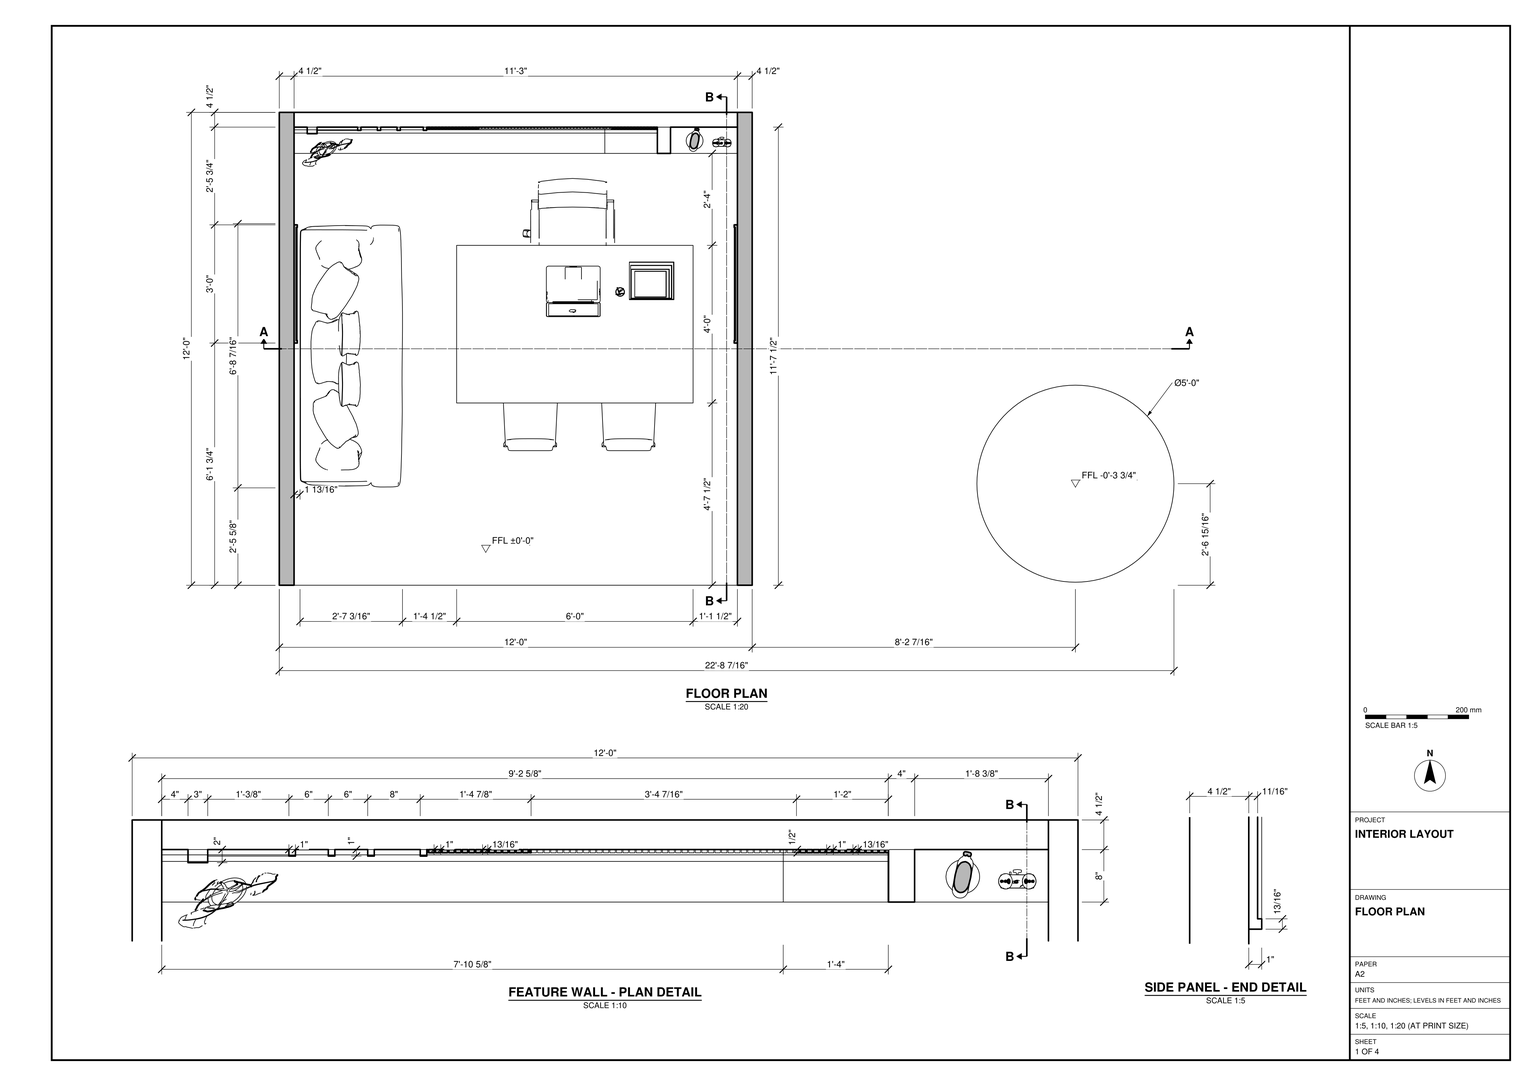
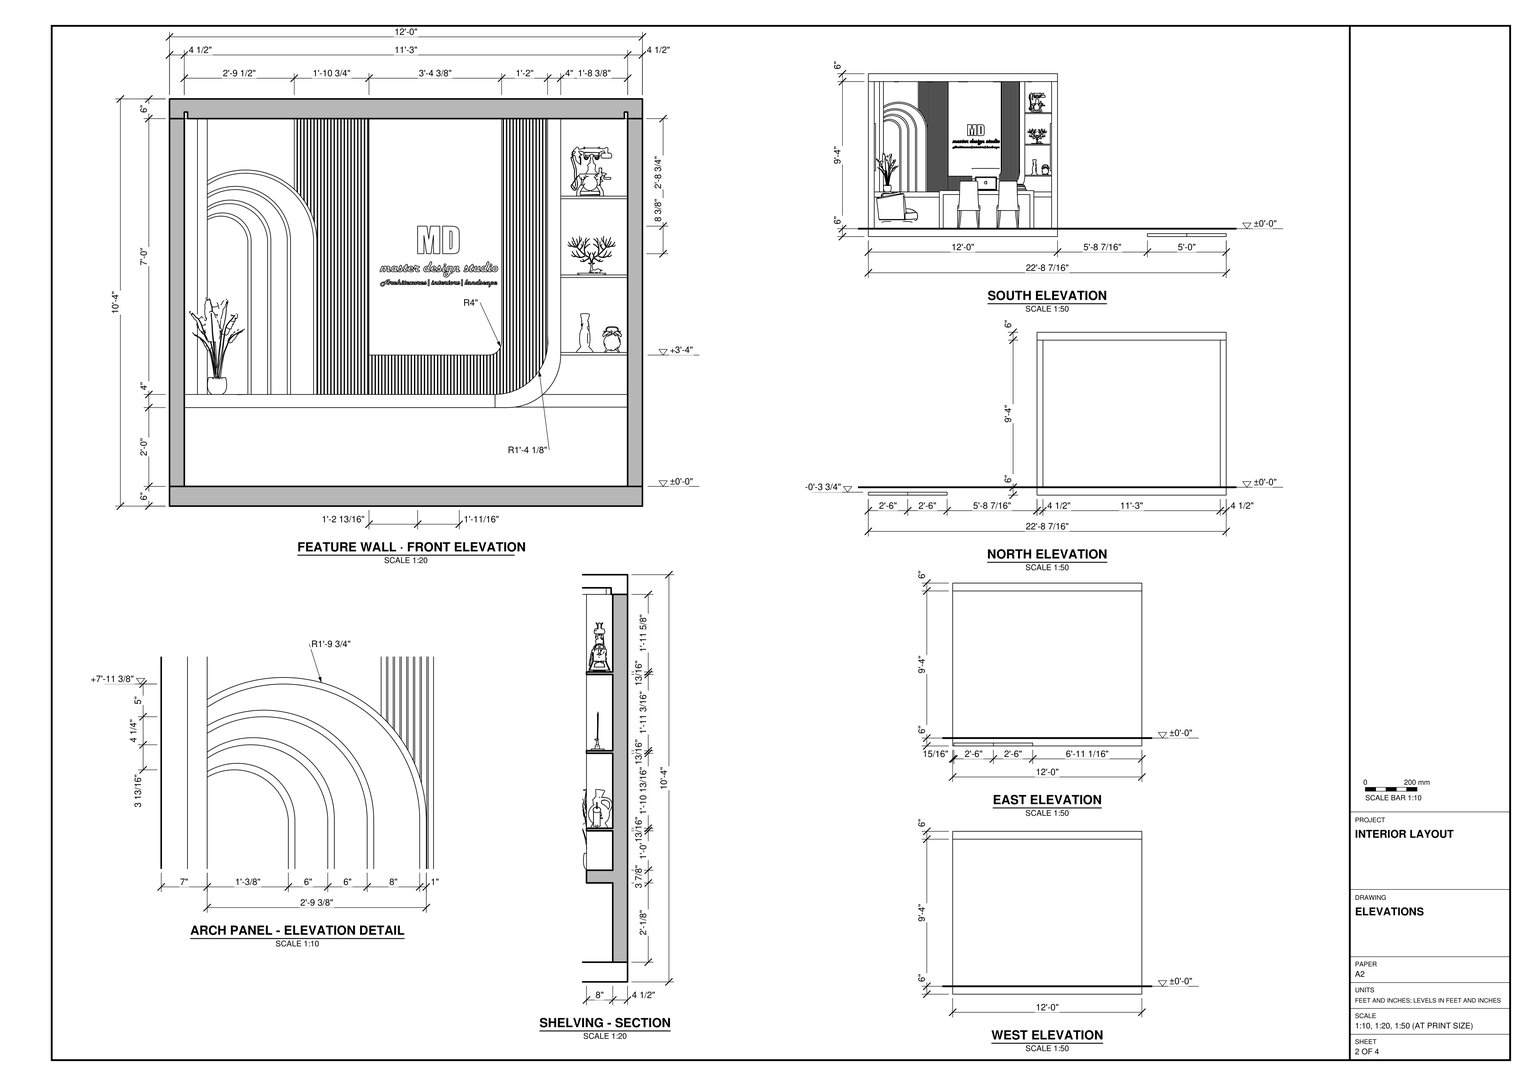
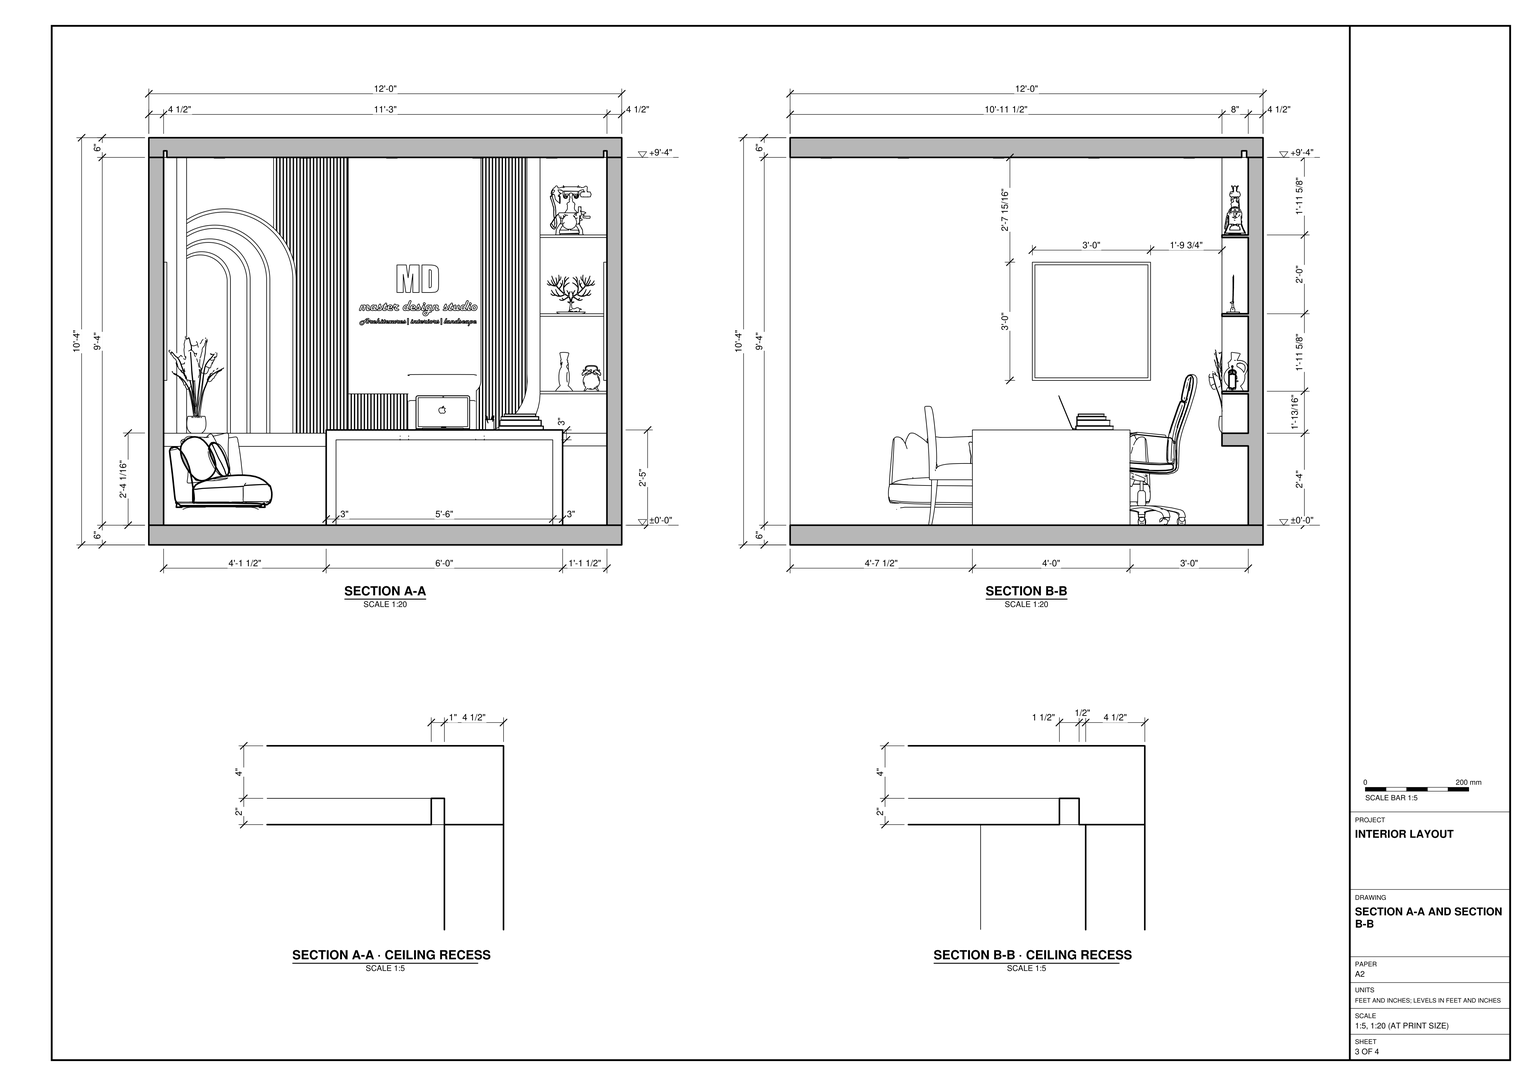
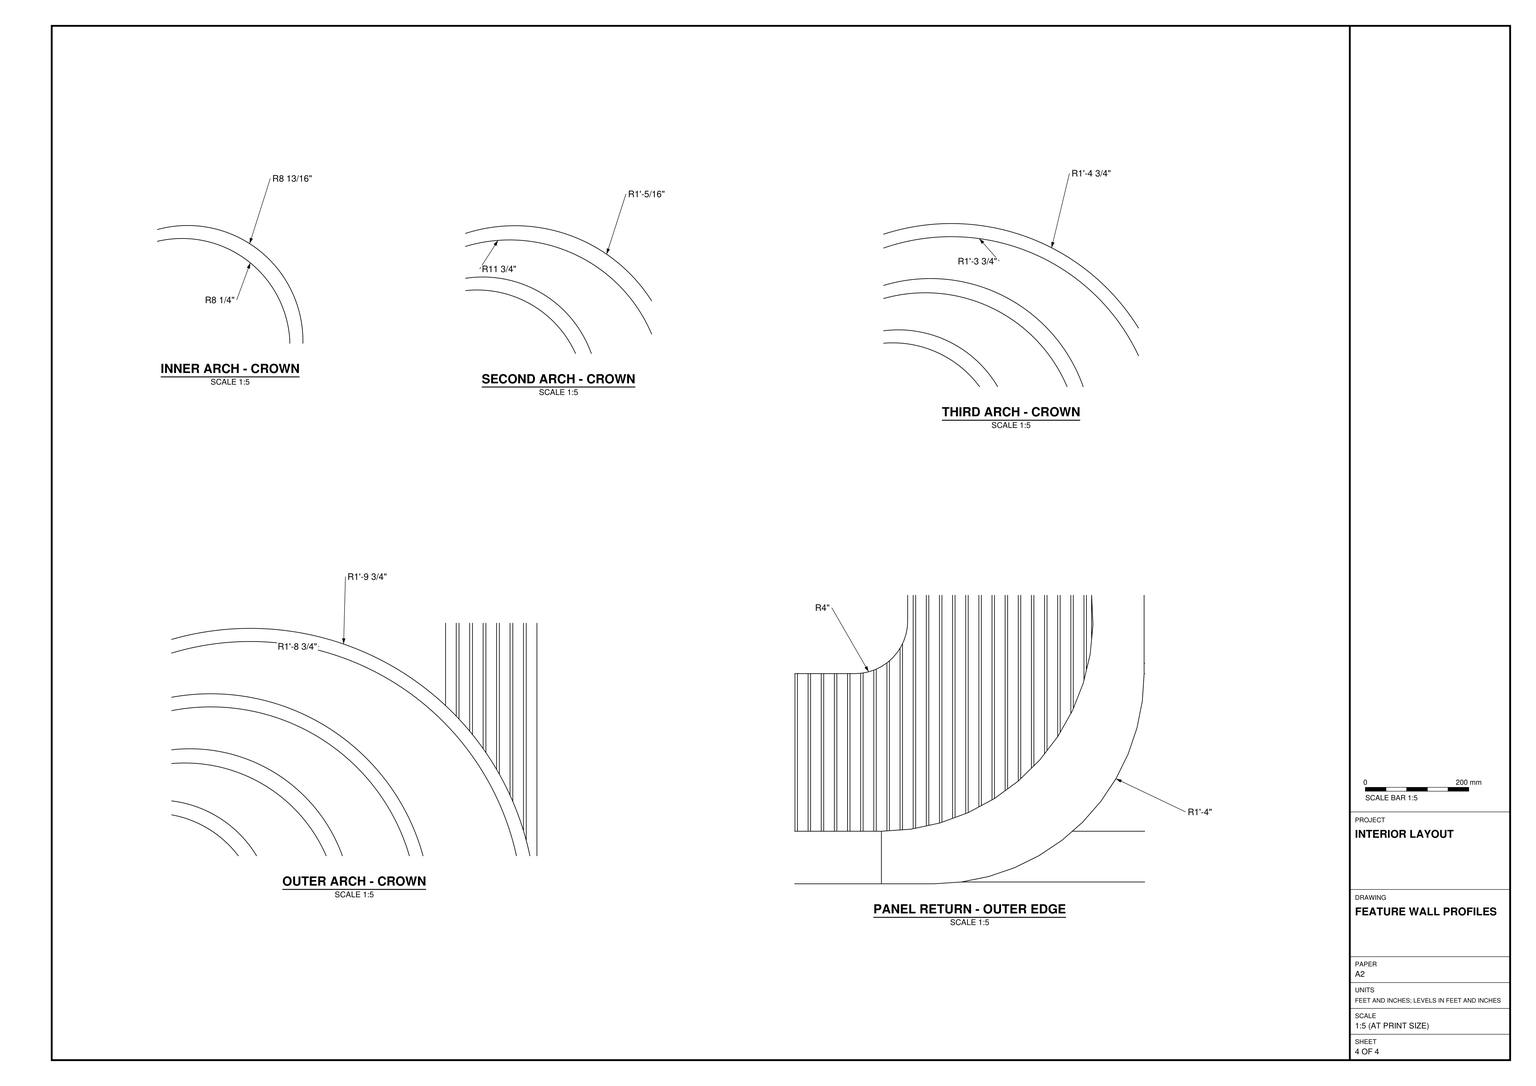
Build the office interior in SketchUp from task_files/diagram_01.pdf. Work in feet and inches. The complete layout measures 22'-8 7/16" across, 12'-0" deep and 10'-4" high. Set the office finished floor at ±0'-0". The room itself has a 12'-0" square footprint; the separate low circular element to its right accounts for the additional width. Use the plan and elevations to place that element at the indicated offset and height.

Leave the front of the office open. Model the 4 1/2" side and back walls, the 6" floor and ceiling slabs, and the narrow ceiling recesses shown in section. Across the back wall, build the raised ledge, nested arch bands, vertical slats, central lettering panel with its rounded lower corner, and open display shelves. Follow the plan detail for the projections of these pieces. Include the square panels on the side walls.

Place the rectangular desk with slab end supports opposite the feature wall, with the office chair between the desk and wall and two visitor chairs facing it. Set the sofa lengthwise along the left wall. Decor and loose items on the ledge, shelves, desk and sofa may be any suitable library components. Keep the walls, slabs, built-in joinery and individual furniture pieces in separate groups or components, and use components for repeated parts. Save one SketchUp model as output_files/furnished_office_with_an_arched_feature_wall.skp.

# SketchUp Ruby script. Lengths in inches.
U = 1.inch
M = Sketchup.active_model
def pt(a) = Geom::Point3d.new(a.map { |v| v * U })
def face(e, loops, mat)
  f = e.add_face(loops[0].map { |a| pt(a) })
  loops[1..].each { |l| e.add_face(l.map { |a| pt(a) }).erase! }
  f.material = f.back_material = mat if mat
  f
end
# faces: each face lists its corners as indices into pts; further lists are holes
def faces(e, pts, list, mat = nil) = list.each { |f| face(e, (f[0].is_a?(Array) ? f : [f]).map { |l| l.map { |i| pts[i] } }, mat) }
# xy, xz, yz: faces in a plane at the given z, y or x. An outline is a flat list of corners, or four numbers for a rectangle; further outlines are holes
def ring(l) = l.size == 4 ? [[l[0], l[1]], [l[2], l[1]], [l[2], l[3]], [l[0], l[3]]] : l.each_slice(2).to_a
def flat(e, list, mat, &to3) = list.each { |f| face(e, (f[0].is_a?(Array) ? f : [f]).map { |l| ring(l).map { |u, v| to3.(u, v) } }, mat) }
def xy(e, z, list, mat = nil) = flat(e, list, mat) { |x, y| [x, y, z] }
def xz(e, y, list, mat = nil) = flat(e, list, mat) { |x, z| [x, y, z] }
def yz(e, x, list, mat = nil) = flat(e, list, mat) { |y, z| [x, y, z] }
def lines(e, pts, list) = list.each { |a, b| e.add_line(pt(pts[a]), pt(pts[b])) }
# prism: a flat outline (further loops are holes) pulled along v
def prism(e, loops, v, mat = nil)
  f = face(e, loops, mat); d = Geom::Vector3d.new(v.map { |x| x * U })
  f.pushpull(f.normal.samedirection?(d) ? d.length : -d.length)
end
def box(e, o, s, mat = nil) = prism(e, [[o, [o[0] + s[0], o[1], o[2]], [o[0] + s[0], o[1] + s[1], o[2]], [o[0], o[1] + s[1], o[2]]]], [0, 0, s[2]], mat)
def at(x, y, z, deg = 0) = Geom::Transformation.translation(pt([x, y, z])) * Geom::Transformation.rotation(ORIGIN, Z_AXIS, deg.degrees)
def axes(o, x, y, z) = Geom::Transformation.new([*x, 0, *y, 0, *z, 0, *pt(o).to_a, 1])
def part(name) = M.definitions.add(name)
# library, detail: a bought-in or finely detailed component or shape, given as its bounding box
def library(name, o, s) = part(name).tap { |d| box(d.entities, o, s) }
def detail(e, o, s) = box(e.add_group.entities, o, s)
def put(e, d, t, mat = nil) = e.add_instance(d, t).tap { |i| i.material = mat if mat }
def group(e, t, mat = nil) = e.add_group.tap { |g| g.transformation = t; g.material = mat if mat }.entities
root = M.entities
M.materials.add("Oak Veneered MDF (Z8GPD2)").color = [209, 167, 120]
M.materials.add("POT_TEXTURE_1").color = [172, 172, 172]
M.materials.add("Teddy_Brim").color = [225, 210, 185]
M.materials.add("[Color M00]").color = [255, 255, 255]
M.materials.add("[Color M00]1").color = [255, 255, 255]
M.materials.add("[Color M09]").color = [0, 0, 0]
M.materials.add("[Color_000]").color = [255, 255, 255]
M.materials.add("[Color_D05]1").color = [255, 242, 204]
M.materials.add("soil1").color = [68, 55, 47]
c1 = part("MD")
prism(c1.entities,[[[3.42,4,0],[3.42,0,0],[2.51,0,0],[2.51,2.7,0],[2.14,0,0],[1.5,0,0],[1.12,2.64,0],[1.12,0,0],[0.21,0,0],[0.21,4,0],[1.55,4,0],[1.68,3.15,0],[1.82,2.13,0],[2.0625,4,0]]],[0,0,2])
prism(c1.entities,[[[3.83,4,0],[4.61,4,0],[5.24,3.98,0],[5.63,3.93,0],[5.87,3.84,0],[6.04,3.7,0],[6.15,3.54,0],[6.21,3.35,0],[6.24,2.59,0],[6.24,1.1875,0],[6.23,0.74,0],[6.19,0.47,0],[6.125,0.31,0],[6.02,0.18,0],[5.875,0.1,0],[5.7,0.04,0],[5.15,0,0],[3.83,0,0]],[[4.875,3.32,0],[4.875,0.68,0],[5.06,0.71,0],[5.15,0.77,0],[5.19,0.94,0],[5.2,1.26,0],[5.2,2.82,0],[5.1875,3.17,0],[5.11,3.28,0]]],[0,0,2])
c2 = library("master design st",[0.17,0,0],[35.89,4.7,2])
c3 = library("Architexures|int",[-0.02,0,0],[30.58,2.32,2])
c4 = library("chairs office (2)",[-15.11,-13.4,-0.04],[27.95,30.25,45.94])
c5 = library("silla generica",[-12.64,0.67,0],[23.23,30.27,48.95])
c6 = library("sofaD71839)",[0.35,-39.08,0.31],[80.46,34.29,30.24])
c7 = library("laptop",[-0.05,16.1,0.9],[15.46,16.39,10.55])
c8 = library("Group\#92",[-662.41,217.3,320.04],[397.32,658.3,1732.06])
c9 = library("Group\#94",[-299.2,181.55,262.58],[360.65,735.71,1258.34])
c10 = library("Group\#89",[-1038.76,656.55,345.34],[733.18,460.51,2065.7])
c11 = library("Group\#87",[-445.29,890.31,329.28],[284.3,304.08,2023.29])
c12 = library("Group\#90",[-733.48,439.625,202.64],[456.28,533.12,1536.78])
c13 = library("Group\#93",[-455.56,899.32,410.78],[341.21,610.33,1581.5])
c14 = library("Group\#86",[-516.34,626.77,-4.5625],[517.73,515.95,418.98])
c15 = library("Group\#91",[-249.24,914.85,310.18],[345.55,647.95,1307.93])
c16 = library("Group\#88",[-277.97,488.68,287.26],[362.84,405.94,1768.54])
c17 = library("Group\#85",[-468.76,669.89,380.1875],[424.36,427.47,41.99])
c18 = part("Potted plant")
put(c18.entities,c8,at(1038.76,-181.55,4.5625))
put(c18.entities,c9,at(1038.76,-181.55,4.5625))
put(c18.entities,c10,at(1038.76,-181.55,4.5625))
put(c18.entities,c11,at(1038.76,-181.55,4.5625))
put(c18.entities,c12,at(1038.76,-181.55,4.5625))
put(c18.entities,c13,at(1038.76,-181.55,4.5625))
put(c18.entities,c14,at(1038.76,-181.55,4.5625),"POT_TEXTURE_1")
put(c18.entities,c15,at(1038.76,-181.55,4.5625))
put(c18.entities,c16,at(1038.76,-181.55,4.5625))
put(c18.entities,c17,at(1038.76,-181.55,4.5625),"soil1")
c19 = library("Telephone 194 013",[-6.23,-3.22,0.01],[12.47,6.44,15])
c20 = library("Decorative Deer 97-30",[-7.23,-2.03,0],[14.46,4,11.8125])
c21 = library("Alarm Clock 114 007",[-2.86,-1.17,0.01],[5.71,2.99,7.86])
c22 = library("Interior Props 221 030",[-2.57,-3.63,-0.04],[5.13,7.27,11.89])
c23 = part("Closed book \#1")
xy(c23.entities,0,[[0.12,0.12,1.66,6.72]])
xy(c23.entities,0,[[0,0,0,6.8,0.12,6.8,0.12,0.12,1.66,0.12,1.66,6.8,1.77,6.8,1.77,0]],"[Color_000]")
xy(c23.entities,9.22,[[0.12,0.12,1.66,6.72]],"[Color_D05]1")
xy(c23.entities,9.33,[[0,0,1.77,0,1.77,6.8,1.66,6.8,1.66,0.12,0.12,0.12,0.12,6.8,0,6.8]],"[Color_000]")
xz(c23.entities,0,[[0,0,1.77,9.33]])
xz(c23.entities,0.12,[[0.12,0,1.66,9.22]])
xz(c23.entities,0.12,[[0.12,9.22,1.66,9.33]],"[Color_000]")
xz(c23.entities,6.72,[[0.12,0,1.66,9.22]],"[Color_D05]1")
xz(c23.entities,6.8,[[0,0,0.12,9.33],[1.66,0,1.77,9.33]],"[Color_000]")
yz(c23.entities,0,[[0,0,6.8,9.33]])
yz(c23.entities,0.12,[[0.12,0,6.72,9.22]])
yz(c23.entities,0.12,[[6.72,0,6.8,0,6.8,9.33,0.12,9.33,0.12,9.22,6.72,9.22]],"[Color_000]")
yz(c23.entities,1.66,[[0.12,0,6.72,9.22]])
yz(c23.entities,1.66,[[6.72,0,6.72,9.22,0.12,9.22,0.12,9.33,6.8,9.33,6.8,0]],"[Color_000]")
yz(c23.entities,1.77,[[0,0,6.8,9.33]])
c24 = part("Closed book \#2")
xy(c24.entities,0,[[0.12,0.12,1.11,7.59]])
xy(c24.entities,0,[[0,0,0,7.67,0.12,7.67,0.12,0.12,1.11,0.12,1.11,7.67,1.22,7.67,1.22,0]],"[Color_000]")
xy(c24.entities,10.875,[[0.12,0.12,1.11,7.59]],"[Color_D05]1")
xy(c24.entities,10.99,[[0,0,1.22,0,1.22,7.67,1.11,7.67,1.11,0.12,0.12,0.12,0.12,7.67,0,7.67]],"[Color_000]")
xz(c24.entities,0,[[0,0,1.22,10.99]])
xz(c24.entities,0.12,[[0.12,0,1.11,10.875]])
xz(c24.entities,0.12,[[0.12,10.875,1.11,10.99]],"[Color_000]")
xz(c24.entities,7.59,[[0.12,0,1.11,10.875]],"[Color_D05]1")
xz(c24.entities,7.67,[[0,0,0.12,10.99]])
xz(c24.entities,7.67,[[1.11,0,1.22,10.99]],"[Color_000]")
yz(c24.entities,0,[[0,0,7.67,10.99]])
yz(c24.entities,0.12,[[0.12,0,7.59,10.875]])
yz(c24.entities,0.12,[[7.59,0,7.67,0,7.67,10.99,0.12,10.99,0.12,10.875,7.59,10.875]],"[Color_000]")
yz(c24.entities,1.11,[[0.12,0,7.59,10.875]])
yz(c24.entities,1.11,[[7.59,0,7.59,10.875,0.12,10.875,0.12,10.99,7.67,10.99,7.67,0]],"[Color_000]")
yz(c24.entities,1.22,[[0,0,7.67,10.99]])
c25 = part("Closed book")
xy(c25.entities,0,[[0.12,0.12,0.99,5.93]])
xy(c25.entities,0,[[0,0,0,6.01,0.12,6.01,0.12,0.12,0.99,0.12,0.99,6.01,1.1,6.01,1.1,0]],"[Color_000]")
xy(c25.entities,9.5,[[0.12,0.12,0.99,5.93]],"[Color_D05]1")
xy(c25.entities,9.61,[[0,0,1.1,0,1.1,6.01,0.99,6.01,0.99,0.12,0.12,0.12,0.12,6.01,0,6.01]],"[Color_000]")
xz(c25.entities,0,[[0,0,1.1,4.45],[0,4.45,1.1,9.61]])
xz(c25.entities,0.12,[[0.12,0,0.99,9.5]])
xz(c25.entities,0.12,[[0.12,9.5,0.99,9.61]],"[Color_000]")
xz(c25.entities,5.93,[[0.12,0,0.99,9.5]],"[Color_D05]1")
xz(c25.entities,6.01,[[0,0,0.12,9.61],[0.99,0,1.1,9.61]],"[Color_000]")
yz(c25.entities,0,[[0,0,6.01,9.61]])
yz(c25.entities,0.12,[[0.12,0,5.93,9.5]])
yz(c25.entities,0.12,[[5.93,0,6.01,0,6.01,9.61,0.12,9.61,0.12,9.5,5.93,9.5]],"[Color_000]")
yz(c25.entities,0.99,[[0.12,0,5.93,9.5]])
yz(c25.entities,0.99,[[5.93,0,5.93,9.5,0.12,9.5,0.12,9.61,6.01,9.61,6.01,0]],"[Color_000]")
yz(c25.entities,1.1,[[0,0,6.01,9.61]])
c26 = part("Closed book \#3")
xy(c26.entities,0,[[0.12,0.12,0.68,7.875]])
xy(c26.entities,0,[[0,0,0,7.95,0.12,7.95,0.12,0.12,0.68,0.12,0.68,7.95,0.79,7.95,0.79,0]],"[Color_000]")
xy(c26.entities,9.5,[[0.12,0.12,0.68,7.875]],"[Color_D05]1")
xy(c26.entities,9.61,[[0,0,0.79,0,0.79,7.95,0.68,7.95,0.68,0.12,0.12,0.12,0.12,7.95,0,7.95]],"[Color_000]")
xz(c26.entities,0,[[0,0,0.79,9.61]])
xz(c26.entities,0.12,[[0.12,0,0.68,9.5]])
xz(c26.entities,0.12,[[0.12,9.5,0.68,9.61]],"[Color_000]")
xz(c26.entities,7.875,[[0.12,0,0.68,9.5]],"[Color_D05]1")
xz(c26.entities,7.95,[[0,0,0.12,9.61],[0.68,0,0.79,9.61]],"[Color_000]")
yz(c26.entities,0,[[0,0,7.95,9.61]])
yz(c26.entities,0.12,[[0.12,0,7.875,9.5]])
yz(c26.entities,0.12,[[7.875,0,7.95,0,7.95,9.61,0.12,9.61,0.12,9.5,7.875,9.5]],"[Color_000]")
yz(c26.entities,0.68,[[0.12,0,7.875,9.5]])
yz(c26.entities,0.68,[[7.875,0,7.875,9.5,0.12,9.5,0.12,9.61,7.95,9.61,7.95,0]],"[Color_000]")
yz(c26.entities,0.79,[[0,0,7.95,9.61]])
c27 = part("Stack of books")
put(c27.entities,c23,axes([0.4,0.3125,3],[0,0,-1],[0,1.5,0],[1.344,0,0]))
put(c27.entities,c24,axes([0,0,1.22],[0,0,-1],[0,1.5,0],[1.236,0,0]))
put(c27.entities,c25,axes([0.65,0.3125,4.1],[0,0,-1],[0,1.5,0],[1.2,0,0]))
put(c27.entities,c26,axes([1.65,0.75,4.89],[0,0,-1],[0,1,0],[1,0,0]))
c28 = library("Pen",[0.21,0.93,0.15],[2.77,2.76,4.45])
c29 = library("Group\#2",[0,-8,0],[135,12.5,112])
c30 = part("Group\#159")
xy(c30.entities,12.39,[[[4.45,2.83,4.03,2.88,3.64,3.04,3.3,3.3,3.04,3.64,2.88,4.03,2.83,4.45,2.88,4.87,3.04,5.26,3.3,5.6,3.64,5.86,4.03,6.02,4.45,6.08,4.87,6.02,5.26,5.86,5.6,5.6,5.86,5.26,6.02,4.87,6.08,4.45,6.02,4.03,5.86,3.64,5.6,3.3,5.26,3.04,4.87,2.88],[4.45,3.45,4.71,3.49,4.95,3.59,5.16,3.75,5.3125,3.95,5.41,4.19,5.45,4.45,5.41,4.71,5.3125,4.95,5.16,5.16,4.95,5.3125,4.71,5.41,4.45,5.45,4.19,5.41,3.95,5.3125,3.75,5.16,3.59,4.95,3.49,4.71,3.45,4.45,3.49,4.19,3.59,3.95,3.75,3.75,3.95,3.59,4.19,3.49]]],"[Color M09]")
xy(c30.entities,12.63,[[4.45,2.83,4.87,2.88,5.26,3.04,5.6,3.3,5.86,3.64,6.02,4.03,6.08,4.45,6.02,4.87,5.86,5.26,5.6,5.6,5.26,5.86,4.87,6.02,4.45,6.08,4.03,6.02,3.64,5.86,3.3,5.6,3.04,5.26,2.88,4.87,2.83,4.45,2.88,4.03,3.04,3.64,3.3,3.3,3.64,3.04,4.03,2.88]],"[Color M09]")
p = [[4.45,2.83,12.63],[4.03,2.88,12.63],[4.03,2.88,12.39],[4.45,2.83,12.39],[4.87,2.88,12.63],[4.87,2.88,12.39],
  [3.64,3.04,12.63],[3.64,3.04,12.39],[5.26,3.04,12.63],[5.26,3.04,12.39],[3.3,3.3,12.63],[3.3,3.3,12.39],
  [5.6,3.3,12.63],[5.6,3.3,12.39],[3.04,3.64,12.63],[3.04,3.64,12.39],[5.86,3.64,12.63],[5.86,3.64,12.39],
  [4.19,3.49,12.39],[3.95,3.59,12.39],[3.95,3.59,12.51],[4.19,3.49,12.51],[4.45,3.45,12.39],[4.45,3.45,12.51],
  [4.71,3.49,12.39],[4.71,3.49,12.51],[4.95,3.59,12.39],[4.95,3.59,12.51],[2.88,4.03,12.63],[2.88,4.03,12.39],
  [3.75,3.75,12.39],[3.75,3.75,12.51],[5.16,3.75,12.39],[5.16,3.75,12.51],[6.02,4.03,12.63],[6.02,4.03,12.39],
  [3.59,3.95,12.39],[3.59,3.95,12.51],[5.3125,3.95,12.39],[5.3125,3.95,12.51],[2.83,4.45,12.63],[2.83,4.45,12.39],
  [3.49,4.19,12.39],[3.49,4.19,12.51],[5.41,4.19,12.39],[5.41,4.19,12.51],[6.08,4.45,12.63],[6.08,4.45,12.39],
  [3.45,4.45,12.39],[3.45,4.45,12.51],[5.45,4.45,12.39],[5.45,4.45,12.51],[2.88,4.87,12.63],[2.88,4.87,12.39],
  [3.49,4.71,12.39],[3.49,4.71,12.51],[5.41,4.71,12.39],[5.41,4.71,12.51],[6.02,4.87,12.63],[6.02,4.87,12.39],
  [3.59,4.95,12.39],[3.59,4.95,12.51],[5.3125,4.95,12.39],[5.3125,4.95,12.51],[3.04,5.26,12.63],[3.04,5.26,12.39],
  [3.75,5.16,12.39],[3.75,5.16,12.51],[5.16,5.16,12.39],[5.16,5.16,12.51],[5.86,5.26,12.63],[5.86,5.26,12.39],
  [3.95,5.3125,12.39],[3.95,5.3125,12.51],[4.95,5.3125,12.39],[4.95,5.3125,12.51],[3.3,5.6,12.63],[3.3,5.6,12.39],
  [4.19,5.41,12.39],[4.19,5.41,12.51],[4.71,5.41,12.39],[4.71,5.41,12.51],[5.6,5.6,12.63],[5.6,5.6,12.39],
  [4.45,5.45,12.39],[4.45,5.45,12.51],[3.64,5.86,12.63],[3.64,5.86,12.39],[5.26,5.86,12.63],[5.26,5.86,12.39],
  [4.03,6.02,12.63],[4.03,6.02,12.39],[4.87,6.02,12.63],[4.87,6.02,12.39],[4.45,6.08,12.63],[4.45,6.08,12.39]]
faces(c30.entities,p,[[0,1,2,3],[4,0,3,5],[1,6,7,2],[8,4,5,9],[6,10,11,7],[12,8,9,13],[10,14,15,11],[16,12,13,17],
  [18,19,20,21],[22,18,21,23],[24,22,23,25],[26,24,25,27],[14,28,29,15],[19,30,31,20],[32,26,27,33],[34,16,17,35],
  [30,36,37,31],[38,32,33,39],[28,40,41,29],[36,42,43,37],[44,38,39,45],[46,34,35,47],[42,48,49,43],[50,44,45,51],
  [40,52,53,41],[48,54,55,49],[56,50,51,57],[58,46,47,59],[54,60,61,55],[62,56,57,63],[52,64,65,53],[60,66,67,61],
  [68,62,63,69],[70,58,59,71],[66,72,73,67],[74,68,69,75],[64,76,77,65],[72,78,79,73],[80,74,75,81],[82,70,71,83],
  [78,84,85,79],[84,80,81,85],[76,86,87,77],[88,82,83,89],[86,90,91,87],[92,88,89,93],[90,94,95,91],[94,92,93,95]],"[Color M09]")
g1 = group(c30.entities,at(3.45,3.45,12.51))
xy(g1,0,[[1,0,0.74,0.03,0.5,0.13,0.29,0.29,0.13,0.5,0.03,0.74,0,1,0.03,1.25,0.13,1.49,0.29,1.7,0.5,1.86,0.74,1.96,1,1.99,1.25,1.96,1.49,1.86,1.7,1.7,1.86,1.49,1.96,1.25,1.99,1,1.96,0.74,1.86,0.5,1.7,0.29,1.49,0.13,1.25,0.03]],"[Color M00]1")
prism(root,[[[272.42,30.93,0],[272.36,29.05,0],[272.1875,27.17,0],[271.89,25.31,0],[271.48,23.47,0],[270.96,21.66,0],[270.32,19.89,0],[269.57,18.16,0],[268.71,16.48,0],[267.75,14.85,0],[266.69,13.3,0],[265.54,11.81,0],[264.29,10.39,0],[262.96,9.0625,0],[261.55,7.8125,0],[260.06,6.66,0],[258.5,5.6,0],[256.875,4.64,0],[255.2,3.78,0],[253.47,3.04,0],[251.69,2.4,0],[249.88,1.87,0],[248.05,1.46,0],[246.18,1.17,0],[244.31,0.99,0],[242.42,0.93,0],[240.54,0.99,0],[238.66,1.17,0],[236.8,1.46,0],[234.96,1.87,0],[233.15,2.4,0],[231.38,3.04,0],[229.65,3.78,0],[227.97,4.64,0],[226.35,5.6,0],[224.79,6.66,0],[223.3,7.8125,0],[221.89,9.0625,0],[220.55,10.39,0],[219.31,11.81,0],[218.15,13.3,0],[217.09,14.85,0],[216.13,16.48,0],[215.28,18.16,0],[214.53,19.89,0],[213.89,21.66,0],[213.37,23.47,0],[212.96,25.31,0],[212.66,27.17,0],[212.48,29.05,0],[212.42,30.93,0],[212.48,32.8125,0],[212.66,34.69,0],[212.96,36.55,0],[213.37,38.39,0],[213.89,40.2,0],[214.53,41.97,0],[215.28,43.7,0],[216.13,45.38,0],[217.09,47,0],[218.15,48.5625,0],[219.31,50.05,0],[220.55,51.47,0],[221.89,52.8,0],[223.3,54.05,0],[224.79,55.2,0],[226.35,56.26,0],[227.97,57.22,0],[229.65,58.07,0],[231.38,58.82,0],[233.15,59.46,0],[234.96,59.99,0],[236.8,60.4,0],[238.66,60.69,0],[240.54,60.87,0],[242.42,60.93,0],[244.31,60.87,0],[246.18,60.69,0],[248.05,60.4,0],[249.88,59.99,0],[251.69,59.46,0],[253.47,58.82,0],[255.2,58.07,0],[256.875,57.22,0],[258.5,56.26,0],[260.06,55.2,0],[261.55,54.05,0],[262.96,52.8,0],[264.29,51.47,0],[265.54,50.05,0],[266.69,48.5625,0],[267.75,47,0],[268.71,45.38,0],[269.57,43.7,0],[270.32,41.97,0],[270.96,40.2,0],[271.48,38.39,0],[271.89,36.55,0],[272.1875,34.69,0],[272.36,32.8125,0]]],[0,0,2.25])
put(root,c1,axes([75.12,139.5,76.86],[2.1,0,0],[0,0,2.1],[0,-0.315,0]),"[Color M09]")
put(root,c2,axes([63.92,139.5,69.73],[1,0,0],[0,0,1],[0,-0.29,0]),"[Color M09]")
put(root,c3,axes([64.22,139.5,66.68],[1.1628,0,0],[0,0,1],[0,-0.29,0]),"[Color M09]")
put(root,c4,at(89.32,107.03,6))
put(root,c5,axes([77.21,63.88,6],[0.74,0,0],[0,-0.74,0],[0,0,0.74]))
put(root,c5,axes([107.15,63.88,6],[0.74,0,0],[0,-0.74,0],[0,0,0.74]))
put(root,c6,axes([1.96,29.3,5.69],[0,1,0],[-0.91,0,0],[0,0,1]))
put(root,c7,at(113.8125,81.77,34.1,90))
put(root,c18,axes([4.03,133.62,34],[0.00376,-0.00652,0],[0.01068,0.00617,0],[0,0,0.01233]))
put(root,c19,at(128.44,135.43,94.39))
put(root,c20,at(128.53,134.9375,70.39))
put(root,c21,at(134.76,134.64,46.79))
put(root,c22,at(126.53,135.68,46.79,-11.4))
put(root,c27,at(106.59,86.94,35))
put(root,c28,at(102.22,87.03,34.85))
g2 = group(root,at(0,0,0))
box(g2,[0,0,0],[144,144,6])
g3 = group(root,at(0,0,6))
box(g3,[0,0,0],[4.5,144,112])
put(root,c29,at(4.5,139.5,6),"Teddy_Brim")
g4 = group(root,at(139.5,0,6))
box(g4,[0,0,0],[4.5,144,112])
g5 = group(root,at(54,55.5,6))
xy(g5,0,[[0,0,0,48,3,48,3,31,69,31,69,48,72,48,72,0,69,0,69,12,3,12,3,0]])
xy(g5,26,[[3,0,69,12],[3,31,69,48]])
xy(g5,29,[[0,0,72,48]],"[Color M00]")
xz(g5,0,[[0,0,3,0,3,26,69,26,69,0,72,0,72,29,0,29]],"[Color M00]")
xz(g5,12,[[3,0,69,26]],"Oak Veneered MDF (Z8GPD2)")
xz(g5,31,[[3,0,69,26]],"Oak Veneered MDF (Z8GPD2)")
xz(g5,48,[[0,0,0,29,72,29,72,0,69,0,69,26,3,26,3,0]],"[Color M00]")
yz(g5,0,[[0,0,48,29]],"[Color M00]")
yz(g5,3,[[0,0,12,26],[31,0,48,26]])
yz(g5,69,[[0,0,12,26]])
yz(g5,69,[[31,0,48,26]],"[Color M00]")
yz(g5,72,[[0,0,48,29]],"[Color M00]")
put(root,c30,at(17.05,117.05,105.37))
put(root,c30,at(43.3,117.05,105.37))
put(root,c30,at(69.55,117.05,105.37))
put(root,c30,at(95.8,117.05,105.37))
put(root,c30,at(118.24,117.05,105.37))
put(root,c30,at(118.24,88.05,105.37))
put(root,c30,at(17.05,88.05,105.37))
put(root,c30,at(118.24,59.05,105.37))
put(root,c30,at(17.05,59.05,105.37))
put(root,c30,at(118.24,30.05,105.37))
put(root,c30,at(17.05,30.05,105.37))
put(root,c30,at(118.24,6.55,105.37))
put(root,c30,at(17.05,6.55,105.37))
put(root,c30,at(65.8,6.55,105.37))
put(root,c30,at(92.17,6.55,105.37))
put(root,c30,at(41.67,6.55,105.37))
g6 = group(root,at(4.5,73.75,50.09))
xy(g6,0,[[0,0,0.98,36]])
xy(g6,0.79,[[0.67,0.79,0.98,35.21]])
xy(g6,35.21,[[0.67,0.79,0.98,35.21]])
xy(g6,36,[[0,0,0.98,36]])
xz(g6,0,[[0,0,0.98,36]])
xz(g6,0.79,[[0.67,0.79,0.98,35.21]])
xz(g6,35.21,[[0.67,0.79,0.98,35.21]])
xz(g6,36,[[0,0,0.98,36]])
yz(g6,0,[[0,0,36,36]])
yz(g6,0.67,[[0.79,0.79,35.21,35.21]])
yz(g6,0.98,[[[0,0,36,36],[0.79,0.79,35.21,35.21]]])
g7 = group(root,at(138.52,73.75,50.09))
xy(g7,0,[[0,0,0.98,36]])
xy(g7,0.79,[[0,0.79,0.3125,35.21]])
xy(g7,35.21,[[0,0.79,0.3125,35.21]])
xy(g7,36,[[0,0,0.98,36]])
xz(g7,0,[[0,0,0.98,36]])
xz(g7,0.79,[[0,0.79,0.3125,35.21]])
xz(g7,35.21,[[0,0.79,0.3125,35.21]])
xz(g7,36,[[0,0,0.98,36]])
yz(g7,0,[[[0,0,36,36],[0.79,0.79,35.21,35.21]]])
yz(g7,0.3125,[[0.79,0.79,35.21,35.21]])
yz(g7,0.98,[[0,0,36,36]])
g8 = group(root,at(0,0,118))
xy(g8,0,[[[0,0,144,144],[4.5,0.95,5.5,0.95,5.5,137.5,138.5,137.5,138.5,0.98,139.5,0.98,139.5,139,4.5,139]]])
xy(g8,6,[[0,0,144,144]])
xz(g8,0,[[0,0,144,6]])
xz(g8,0.95,[[4.5,0,5.5,2]])
xz(g8,0.98,[[138.5,0,139.5,2]])
xz(g8,137.5,[[5.5,0,138.5,2]])
xz(g8,139,[[4.5,0,139.5,2]])
xz(g8,144,[[0,0,144,6]])
yz(g8,0,[[0,0,144,6]])
yz(g8,4.5,[[0.95,0,139,2]])
yz(g8,5.5,[[0.95,0,137.5,2]])
yz(g8,138.5,[[0.98,0,137.5,2]])
yz(g8,139.5,[[0.98,0,139,2]])
yz(g8,144,[[0,0,144,6]])
# 1 loose lines left out
g9 = group(g8,at(4.5,0.95,2))
xy(g9,0,[[0,0,1,136.55]])
g10 = group(g8,at(4.5,137.5,2))
xy(g10,0,[[0,0,135,1.5]])
g11 = group(g8,at(138.5,0.98,2))
xy(g11,0,[[0,0,1,136.52]])
